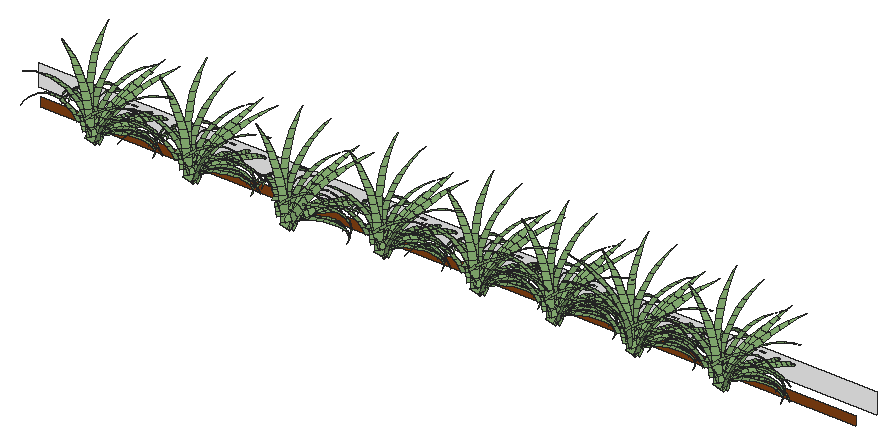
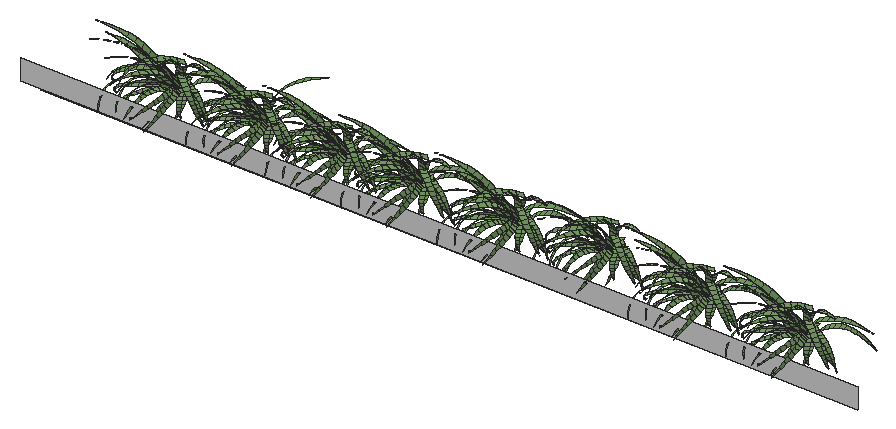
# SketchUp Ruby script. Lengths in inches.
U = 1.inch
M = Sketchup.active_model
def pt(a) = Geom::Point3d.new(a.map { |v| v * U })
def face(e, loops, mat)
  f = e.add_face(loops[0].map { |a| pt(a) })
  loops[1..].each { |l| e.add_face(l.map { |a| pt(a) }).erase! }
  f.material = f.back_material = mat if mat
  f
end
# faces: each face lists its corners as indices into pts; further lists are holes
def faces(e, pts, list, mat = nil) = list.each { |f| face(e, (f[0].is_a?(Array) ? f : [f]).map { |l| l.map { |i| pts[i] } }, mat) }
# xy, xz, yz: faces in a plane at the given z, y or x. An outline is a flat list of corners, or four numbers for a rectangle; further outlines are holes
def ring(l) = l.size == 4 ? [[l[0], l[1]], [l[2], l[1]], [l[2], l[3]], [l[0], l[3]]] : l.each_slice(2).to_a
def flat(e, list, mat, &to3) = list.each { |f| face(e, (f[0].is_a?(Array) ? f : [f]).map { |l| ring(l).map { |u, v| to3.(u, v) } }, mat) }
def xy(e, z, list, mat = nil) = flat(e, list, mat) { |x, y| [x, y, z] }
def xz(e, y, list, mat = nil) = flat(e, list, mat) { |x, z| [x, y, z] }
def yz(e, x, list, mat = nil) = flat(e, list, mat) { |y, z| [x, y, z] }
def lines(e, pts, list) = list.each { |a, b| e.add_line(pt(pts[a]), pt(pts[b])) }
# prism: a flat outline (further loops are holes) pulled along v
def prism(e, loops, v, mat = nil)
  f = face(e, loops, mat); d = Geom::Vector3d.new(v.map { |x| x * U })
  f.pushpull(f.normal.samedirection?(d) ? d.length : -d.length)
end
def box(e, o, s, mat = nil) = prism(e, [[o, [o[0] + s[0], o[1], o[2]], [o[0] + s[0], o[1] + s[1], o[2]], [o[0], o[1] + s[1], o[2]]]], [0, 0, s[2]], mat)
def at(x, y, z, deg = 0) = Geom::Transformation.translation(pt([x, y, z])) * Geom::Transformation.rotation(ORIGIN, Z_AXIS, deg.degrees)
def axes(o, x, y, z) = Geom::Transformation.new([*x, 0, *y, 0, *z, 0, *pt(o).to_a, 1])
def part(name) = M.definitions.add(name)
# library, detail: a bought-in or finely detailed component or shape, given as its bounding box
def library(name, o, s) = part(name).tap { |d| box(d.entities, o, s) }
def detail(e, o, s) = box(e.add_group.entities, o, s)
def put(e, d, t, mat = nil) = e.add_instance(d, t).tap { |i| i.material = mat if mat }
def group(e, t, mat = nil) = e.add_group.tap { |g| g.transformation = t; g.material = mat if mat }.entities
root = M.entities
M.materials.add("[0043_SaddleBrown]").color = [139, 69, 19]
M.materials.add("[Color M00]").color = [255, 255, 255]
M.materials.add("dianella").color = [131, 171, 111]
c1 = part("Shape Bender Component\#7")
p = [[0.01,0.94,1.17],[0.04,0.96,6.32],[0.04,4.67,6.32],[0.01,4.68,1.17],[0.42,0.98,10.52],[0.51,1,11.45],
  [0.51,4.64,11.45],[0.42,4.66,10.52],[1.4,1.07,16.52],[1.4,4.57,16.52],[2.48,1.13,20.62],[2.71,1.16,21.49],
  [2.71,4.49,21.49],[2.48,4.52,20.625],[4.4375,1.21,26.32],[4.4375,4.46,26.32],[6.56,1.22,30.98],[6.56,4.47,30.98],
  [9.06,1.29,35.43],[9.06,4.38,35.43],[11.92,1.42,39.64],[11.92,4.23,39.64],[15.13,1.74,43.57],[15.13,4,43.57],
  [18.65,2.08,47.2],[18.65,3.67,47.2],[22.46,2.47,50.5],[22.46,3.14,50.5],[25.84,2.81,52.95]]
faces(c1.entities,p,[[0,1,2,3],[1,4,5,6,7,2],[5,8,9,6],[10,11,12,13,9,8],[11,14,15,12],[14,16,17,15],[16,18,19,17],[18,20,21,19],
  [20,22,23,21],[22,24,25,23],[24,26,27,25],[28,27,26]],"dianella")
c2 = part("Shape Bender Component\#4")
p = [[0.27,1.78,0.46],[1.95,1.8,3.35],[1.95,4.67,3.35],[0.27,4.68,0.46],[3.06,1.81,4.8],[3.875,1.84,5.87],
  [3.875,4.64,5.87],[3.06,4.66,4.8],[6,1.9,8],[6,4.58,8],[27.35,3.23,6.09],[25.57,3.4375,7.9],
  [25.57,3.03,7.9],[23.28,2.8,9.61],[23.28,3.67,9.61],[7.08,1.93,8.8],[8.3,1.99,9.69],[8.3,4.5,9.69],
  [7.08,4.55,8.8],[23.04,2.78,9.74],[23.04,3.69,9.74],[20.86,3.86,10.86],[20.86,2.625,10.86],[10.73,2.08,10.92],
  [10.73,4.41,10.92],[12.13,2.13,11.33],[13.24,2.19,11.66],[13.24,4.3,11.66],[12.13,4.36,11.33],[18.35,2.46,11.63],
  [18.35,4.03,11.63],[15.79,2.32,11.89],[17.75,2.42,11.69],[17.75,4.07,11.69],[15.79,4.17,11.89]]
faces(c2.entities,p,[[0,1,2,3],[1,4,5,6,7,2],[5,8,9,6],[10,11,12],[13,12,11,14],[15,16,17,18,9,8],[19,13,14,20,21,22],[16,23,24,17],
  [23,25,26,27,28,24],[29,22,21,30],[31,32,29,30,33,34],[26,31,34,27]],"dianella")
c3 = part("Shape Bender Component\#5")
p = [[0.17,0.01,0.72],[1.09,0.03,4.5625],[1.09,3.73,4.5625],[0.17,3.75,0.72],[2.23,0.05,7.59],[2.48,0.0625,8.26],
  [2.48,3.71,8.26],[2.23,3.72,7.59],[4.33,0.14,11.74],[4.33,3.64,11.74],[6.2,0.2,14.41],[6.6,0.22,14.97],
  [6.6,3.56,14.97],[6.2,3.58,14.41],[9.26,0.35,17.88],[9.26,3.43,17.88],[12.27,0.4,20.43],[12.27,3.38,20.43],
  [15.58,0.51,22.59],[15.58,3.27,22.59],[19.13,0.73,24.3],[19.13,3.14,24.3],[22.875,1.08,25.56],[22.875,2.85,25.56],
  [26.75,1.47,26.33],[26.75,2.49,26.33],[30.68,1.86,26.6],[30.68,2.125,26.6],[33.95,1.875,26.45]]
faces(c3.entities,p,[[0,1,2,3],[1,4,5,6,7,2],[5,8,9,6],[8,10,11,12,13,9],[11,14,15,12],[14,16,17,15],[16,18,19,17],[18,20,21,19],
  [20,22,23,21],[22,24,25,23],[24,26,27,25],[28,27,26]],"dianella")
xz(root,570,[[30,281.8125,450,286.25]],"[0043_SaddleBrown]")
xz(root,576,[[24,286.25,456,297.0625]],"[Color M00]")
put(root,c1,axes([351.64,546.07,292.41],[-0.96457,-0.17955,-0.21457],[-0.1415,0.96983,-0.21622],[-0.14686,0.09469,0.71579]))
put(root,c2,axes([116.66,547.22,296.58],[-0.96457,-0.17955,-0.21457],[-0.12461,0.95587,-0.29533],[-0.20696,0.20696,0.93295]))
put(root,c2,axes([215.07,547.22,296.58],[-0.96457,-0.17955,-0.21457],[-0.12461,0.95587,-0.29533],[-0.20696,0.20696,0.93295]))
put(root,c2,axes([303.54,547.22,296.58],[-0.96457,-0.17955,-0.21457],[-0.12461,0.95587,-0.29533],[-0.20696,0.20696,0.93295]))
put(root,c2,axes([389.75,547.22,296.58],[-0.96457,-0.17955,-0.21457],[-0.12461,0.95587,-0.29533],[-0.20696,0.20696,0.93295]))
put(root,c2,axes([66.14,547.22,296.58],[-0.96457,-0.17955,-0.21457],[-0.12461,0.95587,-0.29533],[-0.20696,0.20696,0.93295]))
put(root,c2,axes([264.63,547.22,296.58],[-0.96457,-0.17955,-0.21457],[-0.12461,0.95587,-0.29533],[-0.20696,0.20696,0.93295]))
put(root,c2,axes([344.64,547.22,296.58],[-0.96457,-0.17955,-0.21457],[-0.12461,0.95587,-0.29533],[-0.20696,0.20696,0.93295]))
put(root,c2,axes([180,535.97,302.54],[0.64426,0.58365,-0.4226],[-0.74526,0.62305,-0.21648],[0.16818,0.5202,0.75394]))
put(root,c3,axes([122.69,550.63,289.92],[0.94077,-0.2561,-0.22218],[0.2011,0.94909,-0.24247],[0.24294,0.16325,0.84049]))
put(root,c3,axes([221.1,550.63,289.92],[0.94077,-0.2561,-0.22218],[0.2011,0.94909,-0.24247],[0.24294,0.16325,0.84049]))
put(root,c3,axes([309.57,550.63,289.92],[0.94077,-0.2561,-0.22218],[0.2011,0.94909,-0.24247],[0.24294,0.16325,0.84049]))
put(root,c3,axes([395.78,550.63,289.92],[0.94077,-0.2561,-0.22218],[0.2011,0.94909,-0.24247],[0.24294,0.16325,0.84049]))
put(root,c3,axes([72.17,550.63,289.92],[0.94077,-0.2561,-0.22218],[0.2011,0.94909,-0.24247],[0.24294,0.16325,0.84049]))
put(root,c3,axes([270.66,550.63,289.92],[0.94077,-0.2561,-0.22218],[0.2011,0.94909,-0.24247],[0.24294,0.16325,0.84049]))
put(root,c3,axes([350.67,550.63,289.92],[0.94077,-0.2561,-0.22218],[0.2011,0.94909,-0.24247],[0.24294,0.16325,0.84049]))
put(root,c2,axes([184.96,543.86,301.61],[0.57501,0.09261,-0.46633],[-0.47395,0.84751,-0.13449],[0.65517,0.51591,0.262]))
put(root,c3,axes([123.37,548.09,291.63],[-0.97248,-0.07019,-0.24662],[-0.01462,0.97005,-0.26914],[-0.20696,0.20696,0.93295]))
put(root,c3,axes([221.77,548.09,291.63],[-0.97248,-0.07019,-0.24662],[-0.01462,0.97005,-0.26914],[-0.20696,0.20696,0.93295]))
put(root,c3,axes([310.25,548.09,291.63],[-0.97248,-0.07019,-0.24662],[-0.01462,0.97005,-0.26914],[-0.20696,0.20696,0.93295]))
put(root,c3,axes([396.45,548.09,291.63],[-0.97248,-0.07019,-0.24662],[-0.01462,0.97005,-0.26914],[-0.20696,0.20696,0.93295]))
put(root,c3,axes([72.84,548.09,291.63],[-0.97248,-0.07019,-0.24662],[-0.01462,0.97005,-0.26914],[-0.20696,0.20696,0.93295]))
put(root,c3,axes([271.33,548.09,291.63],[-0.97248,-0.07019,-0.24662],[-0.01462,0.97005,-0.26914],[-0.20696,0.20696,0.93295]))
put(root,c3,axes([351.34,548.09,291.63],[-0.97248,-0.07019,-0.24662],[-0.01462,0.97005,-0.26914],[-0.20696,0.20696,0.93295]))
put(root,c2,axes([183.52,544.4,294.32],[0.57501,0.09261,-0.31801],[-0.47395,0.84751,-0.09172],[0.65517,0.51591,0.17867]))
put(root,c1,axes([175.95,540.82,291.04],[-0.8536,0.41658,-0.34718],[0.46614,0.87885,-0.1128],[-0.15322,0.15322,0.69068]))
put(root,c2,axes([171.79,543.85,295.76],[-0.8536,0.41658,-0.34718],[0.46614,0.87885,-0.1128],[-0.20696,0.20696,0.93295]))
put(root,c2,axes([168.27,544.69,300.99],[-0.54643,0.20158,-0.353],[0.62824,0.74041,-0.10181],[-0.54359,0.63239,0.19832]))
put(root,c2,axes([173.8125,539.64,293.97],[-0.37814,0.80953,-0.24696],[0.77879,0.53846,0.16717],[-0.48914,0.20852,0.40507]))
put(root,c2,axes([182.12,541.8,293.25],[0.43451,0.44271,-0.29722],[-0.79952,0.58659,-0.03391],[0.39557,0.673,0.20362]))
put(root,c3,axes([126.78,546.74,291.2],[0.98276,0.1646,0.08419],[-0.14484,0.96332,-0.19265],[-0.10945,0.21065,0.86584]))
put(root,c3,axes([225.1875,546.74,291.2],[0.98276,0.1646,0.08419],[-0.14484,0.96332,-0.19265],[-0.10945,0.21065,0.86584]))
put(root,c3,axes([313.66,546.74,291.2],[0.98276,0.1646,0.08419],[-0.14484,0.96332,-0.19265],[-0.10945,0.21065,0.86584]))
put(root,c3,axes([399.87,546.74,291.2],[0.98276,0.1646,0.08419],[-0.14484,0.96332,-0.19265],[-0.10945,0.21065,0.86584]))
put(root,c3,axes([76.26,546.74,291.2],[0.98276,0.1646,0.08419],[-0.14484,0.96332,-0.19265],[-0.10945,0.21065,0.86584]))
put(root,c3,axes([274.75,546.74,291.2],[0.98276,0.1646,0.08419],[-0.14484,0.96332,-0.19265],[-0.10945,0.21065,0.86584]))
put(root,c3,axes([354.76,546.74,291.2],[0.98276,0.1646,0.08419],[-0.14484,0.96332,-0.19265],[-0.10945,0.21065,0.86584]))
put(root,c2,axes([127.29,547.1,293.64],[0.91783,0.24445,-0.31277],[-0.28823,0.95215,-0.10163],[0.24294,0.16325,0.84049]))
put(root,c2,axes([225.69,547.1,293.64],[0.91783,0.24445,-0.31277],[-0.28823,0.95215,-0.10163],[0.24294,0.16325,0.84049]))
put(root,c2,axes([314.17,547.1,293.64],[0.91783,0.24445,-0.31277],[-0.28823,0.95215,-0.10163],[0.24294,0.16325,0.84049]))
put(root,c2,axes([400.37,547.1,293.64],[0.91783,0.24445,-0.31277],[-0.28823,0.95215,-0.10163],[0.24294,0.16325,0.84049]))
put(root,c2,axes([76.77,547.1,293.64],[0.91783,0.24445,-0.31277],[-0.28823,0.95215,-0.10163],[0.24294,0.16325,0.84049]))
put(root,c2,axes([275.25,547.1,293.64],[0.91783,0.24445,-0.31277],[-0.28823,0.95215,-0.10163],[0.24294,0.16325,0.84049]))
put(root,c2,axes([355.26,547.1,293.64],[0.91783,0.24445,-0.31277],[-0.28823,0.95215,-0.10163],[0.24294,0.16325,0.84049]))
put(root,c2,axes([169.14,541.87,299.79],[-0.34116,0.51808,-0.32991],[0.89749,0.4217,-0.03764],[-0.25861,0.73656,0.22602]))
put(root,c2,axes([125.52,541.97,302.54],[0.64426,0.58365,-0.4226],[-0.74526,0.62305,-0.21648],[0.16818,0.5202,0.75394]))
put(root,c2,axes([223.92,541.97,302.54],[0.64426,0.58365,-0.4226],[-0.74526,0.62305,-0.21648],[0.16818,0.5202,0.75394]))
put(root,c2,axes([312.4,541.97,302.54],[0.64426,0.58365,-0.4226],[-0.74526,0.62305,-0.21648],[0.16818,0.5202,0.75394]))
put(root,c2,axes([398.6,541.97,302.54],[0.64426,0.58365,-0.4226],[-0.74526,0.62305,-0.21648],[0.16818,0.5202,0.75394]))
put(root,c2,axes([75,541.97,302.54],[0.64426,0.58365,-0.4226],[-0.74526,0.62305,-0.21648],[0.16818,0.5202,0.75394]))
put(root,c2,axes([273.48,541.97,302.54],[0.64426,0.58365,-0.4226],[-0.74526,0.62305,-0.21648],[0.16818,0.5202,0.75394]))
put(root,c2,axes([353.49,541.97,302.54],[0.64426,0.58365,-0.4226],[-0.74526,0.62305,-0.21648],[0.16818,0.5202,0.75394]))
put(root,c2,axes([169.1875,547.18,304.6],[-0.54643,0.20158,-0.51762],[0.62824,0.74041,-0.14929],[-0.54359,0.63239,0.29082]))
put(root,c2,axes([178.9,541.9,290.9375],[0.19337,0.9127,-0.35512],[-0.68492,0.38442,0.57846],[0.69138,0.1105,0.59486]))
put(root,c2,axes([130.48,549.86,301.61],[0.57501,0.09261,-0.46633],[-0.47395,0.84751,-0.13449],[0.65517,0.51591,0.262]))
put(root,c2,axes([228.88,549.86,301.61],[0.57501,0.09261,-0.46633],[-0.47395,0.84751,-0.13449],[0.65517,0.51591,0.262]))
put(root,c2,axes([317.36,549.86,301.61],[0.57501,0.09261,-0.46633],[-0.47395,0.84751,-0.13449],[0.65517,0.51591,0.262]))
put(root,c2,axes([403.56,549.86,301.61],[0.57501,0.09261,-0.46633],[-0.47395,0.84751,-0.13449],[0.65517,0.51591,0.262]))
put(root,c2,axes([79.96,549.86,301.61],[0.57501,0.09261,-0.46633],[-0.47395,0.84751,-0.13449],[0.65517,0.51591,0.262]))
put(root,c2,axes([278.44,549.86,301.61],[0.57501,0.09261,-0.46633],[-0.47395,0.84751,-0.13449],[0.65517,0.51591,0.262]))
put(root,c2,axes([358.45,549.86,301.61],[0.57501,0.09261,-0.46633],[-0.47395,0.84751,-0.13449],[0.65517,0.51591,0.262]))
put(root,c2,axes([181.62,542.72,288.01],[0.00951,0.98109,-0.1933],[-0.96198,0.06174,0.26606],[0.24294,0.16325,0.84049]))
put(root,c2,axes([129.04,550.4,294.32],[0.57501,0.09261,-0.31801],[-0.47395,0.84751,-0.09172],[0.65517,0.51591,0.17867]))
put(root,c2,axes([227.44,550.4,294.32],[0.57501,0.09261,-0.31801],[-0.47395,0.84751,-0.09172],[0.65517,0.51591,0.17867]))
put(root,c2,axes([315.92,550.4,294.32],[0.57501,0.09261,-0.31801],[-0.47395,0.84751,-0.09172],[0.65517,0.51591,0.17867]))
put(root,c2,axes([402.125,550.4,294.32],[0.57501,0.09261,-0.31801],[-0.47395,0.84751,-0.09172],[0.65517,0.51591,0.17867]))
put(root,c2,axes([78.52,550.4,294.32],[0.57501,0.09261,-0.31801],[-0.47395,0.84751,-0.09172],[0.65517,0.51591,0.17867]))
put(root,c2,axes([277,550.4,294.32],[0.57501,0.09261,-0.31801],[-0.47395,0.84751,-0.09172],[0.65517,0.51591,0.17867]))
put(root,c2,axes([357.01,550.4,294.32],[0.57501,0.09261,-0.31801],[-0.47395,0.84751,-0.09172],[0.65517,0.51591,0.17867]))
put(root,c1,axes([180.08,542.89,287.55],[0.29029,0.93027,-0.22347],[-0.88563,0.34788,0.30262],[0.28937,0.069,0.69734]))
put(root,c1,axes([121.47,546.82,291.04],[-0.8536,0.41658,-0.34718],[0.46614,0.87885,-0.1128],[-0.15322,0.15322,0.69068]))
put(root,c1,axes([219.87,546.82,291.04],[-0.8536,0.41658,-0.34718],[0.46614,0.87885,-0.1128],[-0.15322,0.15322,0.69068]))
put(root,c1,axes([308.35,546.82,291.04],[-0.8536,0.41658,-0.34718],[0.46614,0.87885,-0.1128],[-0.15322,0.15322,0.69068]))
put(root,c1,axes([394.55,546.82,291.04],[-0.8536,0.41658,-0.34718],[0.46614,0.87885,-0.1128],[-0.15322,0.15322,0.69068]))
put(root,c1,axes([70.95,546.82,291.04],[-0.8536,0.41658,-0.34718],[0.46614,0.87885,-0.1128],[-0.15322,0.15322,0.69068]))
put(root,c1,axes([269.43,546.82,291.04],[-0.8536,0.41658,-0.34718],[0.46614,0.87885,-0.1128],[-0.15322,0.15322,0.69068]))
put(root,c1,axes([349.44,546.82,291.04],[-0.8536,0.41658,-0.34718],[0.46614,0.87885,-0.1128],[-0.15322,0.15322,0.69068]))
put(root,c2,axes([174.76,544.09,292.76],[-0.01403,0.93285,-0.39418],[0.74612,0.24536,0.64209],[-0.65717,0.24154,0.6603]))
put(root,c2,axes([117.3,549.85,295.76],[-0.8536,0.41658,-0.34718],[0.46614,0.87885,-0.1128],[-0.20696,0.20696,0.93295]))
put(root,c2,axes([215.71,549.85,295.76],[-0.8536,0.41658,-0.34718],[0.46614,0.87885,-0.1128],[-0.20696,0.20696,0.93295]))
put(root,c2,axes([304.1875,549.85,295.76],[-0.8536,0.41658,-0.34718],[0.46614,0.87885,-0.1128],[-0.20696,0.20696,0.93295]))
put(root,c2,axes([390.39,549.85,295.76],[-0.8536,0.41658,-0.34718],[0.46614,0.87885,-0.1128],[-0.20696,0.20696,0.93295]))
put(root,c2,axes([66.78,549.85,295.76],[-0.8536,0.41658,-0.34718],[0.46614,0.87885,-0.1128],[-0.20696,0.20696,0.93295]))
put(root,c2,axes([265.27,549.85,295.76],[-0.8536,0.41658,-0.34718],[0.46614,0.87885,-0.1128],[-0.20696,0.20696,0.93295]))
put(root,c2,axes([345.28,549.85,295.76],[-0.8536,0.41658,-0.34718],[0.46614,0.87885,-0.1128],[-0.20696,0.20696,0.93295]))
put(root,c2,axes([113.78,550.69,300.99],[-0.54643,0.20158,-0.353],[0.62824,0.74041,-0.10181],[-0.54359,0.63239,0.19832]))
put(root,c2,axes([212.1875,550.69,300.99],[-0.54643,0.20158,-0.353],[0.62824,0.74041,-0.10181],[-0.54359,0.63239,0.19832]))
put(root,c2,axes([300.66,550.69,300.99],[-0.54643,0.20158,-0.353],[0.62824,0.74041,-0.10181],[-0.54359,0.63239,0.19832]))
put(root,c2,axes([386.87,550.69,300.99],[-0.54643,0.20158,-0.353],[0.62824,0.74041,-0.10181],[-0.54359,0.63239,0.19832]))
put(root,c2,axes([63.26,550.69,300.99],[-0.54643,0.20158,-0.353],[0.62824,0.74041,-0.10181],[-0.54359,0.63239,0.19832]))
put(root,c2,axes([261.75,550.69,300.99],[-0.54643,0.20158,-0.353],[0.62824,0.74041,-0.10181],[-0.54359,0.63239,0.19832]))
put(root,c2,axes([341.76,550.69,300.99],[-0.54643,0.20158,-0.353],[0.62824,0.74041,-0.10181],[-0.54359,0.63239,0.19832]))
put(root,c2,axes([119.33,545.64,293.97],[-0.37814,0.80953,-0.24696],[0.77879,0.53846,0.16717],[-0.48914,0.20852,0.40507]))
put(root,c2,axes([217.73,545.64,293.97],[-0.37814,0.80953,-0.24696],[0.77879,0.53846,0.16717],[-0.48914,0.20852,0.40507]))
put(root,c2,axes([306.21,545.64,293.97],[-0.37814,0.80953,-0.24696],[0.77879,0.53846,0.16717],[-0.48914,0.20852,0.40507]))
put(root,c2,axes([392.41,545.64,293.97],[-0.37814,0.80953,-0.24696],[0.77879,0.53846,0.16717],[-0.48914,0.20852,0.40507]))
put(root,c2,axes([68.81,545.64,293.97],[-0.37814,0.80953,-0.24696],[0.77879,0.53846,0.16717],[-0.48914,0.20852,0.40507]))
put(root,c2,axes([267.29,545.64,293.97],[-0.37814,0.80953,-0.24696],[0.77879,0.53846,0.16717],[-0.48914,0.20852,0.40507]))
put(root,c2,axes([347.3,545.64,293.97],[-0.37814,0.80953,-0.24696],[0.77879,0.53846,0.16717],[-0.48914,0.20852,0.40507]))
put(root,c2,axes([127.63,547.8,293.25],[0.43451,0.44271,-0.29722],[-0.79952,0.58659,-0.03391],[0.39557,0.673,0.20362]))
put(root,c2,axes([226.04,547.8,293.25],[0.43451,0.44271,-0.29722],[-0.79952,0.58659,-0.03391],[0.39557,0.673,0.20362]))
put(root,c2,axes([314.51,547.8,293.25],[0.43451,0.44271,-0.29722],[-0.79952,0.58659,-0.03391],[0.39557,0.673,0.20362]))
put(root,c2,axes([400.72,547.8,293.25],[0.43451,0.44271,-0.29722],[-0.79952,0.58659,-0.03391],[0.39557,0.673,0.20362]))
put(root,c2,axes([77.11,547.8,293.25],[0.43451,0.44271,-0.29722],[-0.79952,0.58659,-0.03391],[0.39557,0.673,0.20362]))
put(root,c2,axes([275.6,547.8,293.25],[0.43451,0.44271,-0.29722],[-0.79952,0.58659,-0.03391],[0.39557,0.673,0.20362]))
put(root,c2,axes([355.61,547.8,293.25],[0.43451,0.44271,-0.29722],[-0.79952,0.58659,-0.03391],[0.39557,0.673,0.20362]))
put(root,c2,axes([183,545.71,291.44],[0.00951,0.98109,-0.1933],[-0.71163,0.13509,0.65066],[0.69138,0.1105,0.59486]))
put(root,c1,axes([181.62,544.44,287.67],[0.00951,0.98109,-0.1933],[-0.96198,0.06174,0.26606],[0.1822,0.12244,0.63037]))
put(root,c2,axes([174.41,546.42,289.51],[0.17955,0.96457,-0.21457],[0.95587,-0.12461,0.29533],[-0.20696,0.20696,0.93295]))
put(root,c2,axes([114.66,547.87,299.79],[-0.34116,0.51808,-0.32991],[0.89749,0.4217,-0.03764],[-0.25861,0.73656,0.22602]))
put(root,c2,axes([213.07,547.87,299.79],[-0.34116,0.51808,-0.32991],[0.89749,0.4217,-0.03764],[-0.25861,0.73656,0.22602]))
put(root,c2,axes([301.54,547.87,299.79],[-0.34116,0.51808,-0.32991],[0.89749,0.4217,-0.03764],[-0.25861,0.73656,0.22602]))
put(root,c2,axes([387.75,547.87,299.79],[-0.34116,0.51808,-0.32991],[0.89749,0.4217,-0.03764],[-0.25861,0.73656,0.22602]))
put(root,c2,axes([64.14,547.87,299.79],[-0.34116,0.51808,-0.32991],[0.89749,0.4217,-0.03764],[-0.25861,0.73656,0.22602]))
put(root,c2,axes([262.625,547.87,299.79],[-0.34116,0.51808,-0.32991],[0.89749,0.4217,-0.03764],[-0.25861,0.73656,0.22602]))
put(root,c2,axes([342.64,547.87,299.79],[-0.34116,0.51808,-0.32991],[0.89749,0.4217,-0.03764],[-0.25861,0.73656,0.22602]))
put(root,c1,axes([173.79,545.28,289],[-0.10576,0.96875,-0.24806],[0.93604,0.17087,0.33591],[-0.27067,0.12342,0.77405]))
put(root,c3,axes([178.19,542.87,288.69],[-0.09945,0.98178,-0.16194],[-0.95687,-0.04972,0.28623],[0.24294,0.16325,0.84049]))
put(root,c2,axes([186.44,547.68,294.24],[0.19337,0.9127,-0.35512],[-0.68492,0.38442,0.57846],[0.69138,0.1105,0.59486]))
put(root,c2,axes([114.7,553.18,304.6],[-0.54643,0.20158,-0.51762],[0.62824,0.74041,-0.14929],[-0.54359,0.63239,0.29082]))
put(root,c2,axes([213.11,553.18,304.6],[-0.54643,0.20158,-0.51762],[0.62824,0.74041,-0.14929],[-0.54359,0.63239,0.29082]))
put(root,c2,axes([301.59,553.18,304.6],[-0.54643,0.20158,-0.51762],[0.62824,0.74041,-0.14929],[-0.54359,0.63239,0.29082]))
put(root,c2,axes([387.79,553.18,304.6],[-0.54643,0.20158,-0.51762],[0.62824,0.74041,-0.14929],[-0.54359,0.63239,0.29082]))
put(root,c2,axes([64.18,553.18,304.6],[-0.54643,0.20158,-0.51762],[0.62824,0.74041,-0.14929],[-0.54359,0.63239,0.29082]))
put(root,c2,axes([262.67,553.18,304.6],[-0.54643,0.20158,-0.51762],[0.62824,0.74041,-0.14929],[-0.54359,0.63239,0.29082]))
put(root,c2,axes([342.68,553.18,304.6],[-0.54643,0.20158,-0.51762],[0.62824,0.74041,-0.14929],[-0.54359,0.63239,0.29082]))
put(root,c2,axes([124.41,547.9,290.9375],[0.19337,0.9127,-0.35512],[-0.68492,0.38442,0.57846],[0.69138,0.1105,0.59486]))
put(root,c2,axes([222.82,547.9,290.9375],[0.19337,0.9127,-0.35512],[-0.68492,0.38442,0.57846],[0.69138,0.1105,0.59486]))
put(root,c2,axes([311.29,547.9,290.9375],[0.19337,0.9127,-0.35512],[-0.68492,0.38442,0.57846],[0.69138,0.1105,0.59486]))
put(root,c2,axes([397.5,547.9,290.9375],[0.19337,0.9127,-0.35512],[-0.68492,0.38442,0.57846],[0.69138,0.1105,0.59486]))
put(root,c2,axes([73.89,547.9,290.9375],[0.19337,0.9127,-0.35512],[-0.68492,0.38442,0.57846],[0.69138,0.1105,0.59486]))
put(root,c2,axes([272.38,547.9,290.9375],[0.19337,0.9127,-0.35512],[-0.68492,0.38442,0.57846],[0.69138,0.1105,0.59486]))
put(root,c2,axes([352.39,547.9,290.9375],[0.19337,0.9127,-0.35512],[-0.68492,0.38442,0.57846],[0.69138,0.1105,0.59486]))
put(root,c3,axes([175.64,544.9,290.26],[0.28661,0.94426,-0.17976],[0.9294,-0.23301,0.31772],[-0.20696,0.20696,0.93295]))
put(root,c2,axes([171.47,548.61,293.3125],[0.17955,0.96457,-0.21457],[0.72432,-0.00444,0.72223],[-0.65717,0.24154,0.6603]))
put(root,c1,axes([172.58,547.1,289.13],[0.17955,0.96457,-0.21457],[0.95587,-0.12461,0.29533],[-0.15522,0.15522,0.69971]))
put(root,c2,axes([127.13,548.72,288.01],[0.00951,0.98109,-0.1933],[-0.96198,0.06174,0.26606],[0.24294,0.16325,0.84049]))
put(root,c2,axes([225.54,548.72,288.01],[0.00951,0.98109,-0.1933],[-0.96198,0.06174,0.26606],[0.24294,0.16325,0.84049]))
put(root,c2,axes([314.02,548.72,288.01],[0.00951,0.98109,-0.1933],[-0.96198,0.06174,0.26606],[0.24294,0.16325,0.84049]))
put(root,c2,axes([400.22,548.72,288.01],[0.00951,0.98109,-0.1933],[-0.96198,0.06174,0.26606],[0.24294,0.16325,0.84049]))
put(root,c2,axes([76.61,548.72,288.01],[0.00951,0.98109,-0.1933],[-0.96198,0.06174,0.26606],[0.24294,0.16325,0.84049]))
put(root,c2,axes([275.1,548.72,288.01],[0.00951,0.98109,-0.1933],[-0.96198,0.06174,0.26606],[0.24294,0.16325,0.84049]))
put(root,c2,axes([355.11,548.72,288.01],[0.00951,0.98109,-0.1933],[-0.96198,0.06174,0.26606],[0.24294,0.16325,0.84049]))
put(root,c1,axes([125.59,548.89,287.55],[0.29029,0.93027,-0.22347],[-0.88563,0.34788,0.30262],[0.28937,0.069,0.69734]))
put(root,c1,axes([224,548.89,287.55],[0.29029,0.93027,-0.22347],[-0.88563,0.34788,0.30262],[0.28937,0.069,0.69734]))
put(root,c1,axes([312.47,548.89,287.55],[0.29029,0.93027,-0.22347],[-0.88563,0.34788,0.30262],[0.28937,0.069,0.69734]))
put(root,c1,axes([398.68,548.89,287.55],[0.29029,0.93027,-0.22347],[-0.88563,0.34788,0.30262],[0.28937,0.069,0.69734]))
put(root,c1,axes([75.07,548.89,287.55],[0.29029,0.93027,-0.22347],[-0.88563,0.34788,0.30262],[0.28937,0.069,0.69734]))
put(root,c1,axes([273.56,548.89,287.55],[0.29029,0.93027,-0.22347],[-0.88563,0.34788,0.30262],[0.28937,0.069,0.69734]))
put(root,c1,axes([353.57,548.89,287.55],[0.29029,0.93027,-0.22347],[-0.88563,0.34788,0.30262],[0.28937,0.069,0.69734]))
put(root,c2,axes([120.28,550.09,292.76],[-0.01403,0.93285,-0.39418],[0.74612,0.24536,0.64209],[-0.65717,0.24154,0.6603]))
put(root,c2,axes([218.68,550.09,292.76],[-0.01403,0.93285,-0.39418],[0.74612,0.24536,0.64209],[-0.65717,0.24154,0.6603]))
put(root,c2,axes([307.16,550.09,292.76],[-0.01403,0.93285,-0.39418],[0.74612,0.24536,0.64209],[-0.65717,0.24154,0.6603]))
put(root,c2,axes([393.36,550.09,292.76],[-0.01403,0.93285,-0.39418],[0.74612,0.24536,0.64209],[-0.65717,0.24154,0.6603]))
put(root,c2,axes([69.76,550.09,292.76],[-0.01403,0.93285,-0.39418],[0.74612,0.24536,0.64209],[-0.65717,0.24154,0.6603]))
put(root,c2,axes([268.24,550.09,292.76],[-0.01403,0.93285,-0.39418],[0.74612,0.24536,0.64209],[-0.65717,0.24154,0.6603]))
put(root,c2,axes([348.25,550.09,292.76],[-0.01403,0.93285,-0.39418],[0.74612,0.24536,0.64209],[-0.65717,0.24154,0.6603]))
put(root,c2,axes([128.52,551.71,291.44],[0.00951,0.98109,-0.1933],[-0.71163,0.13509,0.65066],[0.69138,0.1105,0.59486]))
put(root,c2,axes([226.92,551.71,291.44],[0.00951,0.98109,-0.1933],[-0.71163,0.13509,0.65066],[0.69138,0.1105,0.59486]))
put(root,c2,axes([315.4,551.71,291.44],[0.00951,0.98109,-0.1933],[-0.71163,0.13509,0.65066],[0.69138,0.1105,0.59486]))
put(root,c2,axes([401.6,551.71,291.44],[0.00951,0.98109,-0.1933],[-0.71163,0.13509,0.65066],[0.69138,0.1105,0.59486]))
put(root,c2,axes([77.99,551.71,291.44],[0.00951,0.98109,-0.1933],[-0.71163,0.13509,0.65066],[0.69138,0.1105,0.59486]))
put(root,c2,axes([276.48,551.71,291.44],[0.00951,0.98109,-0.1933],[-0.71163,0.13509,0.65066],[0.69138,0.1105,0.59486]))
put(root,c2,axes([356.49,551.71,291.44],[0.00951,0.98109,-0.1933],[-0.71163,0.13509,0.65066],[0.69138,0.1105,0.59486]))
put(root,c2,axes([168.47,551.21,296.42],[-0.01403,0.93285,-0.39418],[0.74612,0.24536,0.64209],[-0.65717,0.24154,0.6603]))
put(root,c1,axes([127.13,550.44,287.67],[0.00951,0.98109,-0.1933],[-0.96198,0.06174,0.26606],[0.1822,0.12244,0.63037]))
put(root,c1,axes([225.54,550.44,287.67],[0.00951,0.98109,-0.1933],[-0.96198,0.06174,0.26606],[0.1822,0.12244,0.63037]))
put(root,c1,axes([314.01,550.44,287.67],[0.00951,0.98109,-0.1933],[-0.96198,0.06174,0.26606],[0.1822,0.12244,0.63037]))
put(root,c1,axes([400.22,550.44,287.67],[0.00951,0.98109,-0.1933],[-0.96198,0.06174,0.26606],[0.1822,0.12244,0.63037]))
put(root,c1,axes([76.61,550.44,287.67],[0.00951,0.98109,-0.1933],[-0.96198,0.06174,0.26606],[0.1822,0.12244,0.63037]))
put(root,c1,axes([275.1,550.44,287.67],[0.00951,0.98109,-0.1933],[-0.96198,0.06174,0.26606],[0.1822,0.12244,0.63037]))
put(root,c1,axes([355.11,550.44,287.67],[0.00951,0.98109,-0.1933],[-0.96198,0.06174,0.26606],[0.1822,0.12244,0.63037]))
put(root,c2,axes([119.92,552.42,289.51],[0.17955,0.96457,-0.21457],[0.95587,-0.12461,0.29533],[-0.20696,0.20696,0.93295]))
put(root,c2,axes([218.33,552.42,289.51],[0.17955,0.96457,-0.21457],[0.95587,-0.12461,0.29533],[-0.20696,0.20696,0.93295]))
put(root,c2,axes([306.8,552.42,289.51],[0.17955,0.96457,-0.21457],[0.95587,-0.12461,0.29533],[-0.20696,0.20696,0.93295]))
put(root,c2,axes([393.01,552.42,289.51],[0.17955,0.96457,-0.21457],[0.95587,-0.12461,0.29533],[-0.20696,0.20696,0.93295]))
put(root,c2,axes([69.4,552.42,289.51],[0.17955,0.96457,-0.21457],[0.95587,-0.12461,0.29533],[-0.20696,0.20696,0.93295]))
put(root,c2,axes([267.89,552.42,289.51],[0.17955,0.96457,-0.21457],[0.95587,-0.12461,0.29533],[-0.20696,0.20696,0.93295]))
put(root,c2,axes([347.9,552.42,289.51],[0.17955,0.96457,-0.21457],[0.95587,-0.12461,0.29533],[-0.20696,0.20696,0.93295]))
put(root,c1,axes([119.31,551.28,289],[-0.10576,0.96875,-0.24806],[0.93604,0.17087,0.33591],[-0.27067,0.12342,0.77405]))
put(root,c1,axes([217.72,551.28,289],[-0.10576,0.96875,-0.24806],[0.93604,0.17087,0.33591],[-0.27067,0.12342,0.77405]))
put(root,c1,axes([306.19,551.28,289],[-0.10576,0.96875,-0.24806],[0.93604,0.17087,0.33591],[-0.27067,0.12342,0.77405]))
put(root,c1,axes([392.4,551.28,289],[-0.10576,0.96875,-0.24806],[0.93604,0.17087,0.33591],[-0.27067,0.12342,0.77405]))
put(root,c1,axes([68.79,551.28,289],[-0.10576,0.96875,-0.24806],[0.93604,0.17087,0.33591],[-0.27067,0.12342,0.77405]))
put(root,c1,axes([267.28,551.28,289],[-0.10576,0.96875,-0.24806],[0.93604,0.17087,0.33591],[-0.27067,0.12342,0.77405]))
put(root,c1,axes([347.29,551.28,289],[-0.10576,0.96875,-0.24806],[0.93604,0.17087,0.33591],[-0.27067,0.12342,0.77405]))
put(root,c3,axes([123.71,548.87,288.69],[-0.09945,0.98178,-0.16194],[-0.95687,-0.04972,0.28623],[0.24294,0.16325,0.84049]))
put(root,c3,axes([222.11,548.87,288.69],[-0.09945,0.98178,-0.16194],[-0.95687,-0.04972,0.28623],[0.24294,0.16325,0.84049]))
put(root,c3,axes([310.59,548.87,288.69],[-0.09945,0.98178,-0.16194],[-0.95687,-0.04972,0.28623],[0.24294,0.16325,0.84049]))
put(root,c3,axes([396.79,548.87,288.69],[-0.09945,0.98178,-0.16194],[-0.95687,-0.04972,0.28623],[0.24294,0.16325,0.84049]))
put(root,c3,axes([73.1875,548.87,288.69],[-0.09945,0.98178,-0.16194],[-0.95687,-0.04972,0.28623],[0.24294,0.16325,0.84049]))
put(root,c3,axes([271.67,548.87,288.69],[-0.09945,0.98178,-0.16194],[-0.95687,-0.04972,0.28623],[0.24294,0.16325,0.84049]))
put(root,c3,axes([351.68,548.87,288.69],[-0.09945,0.98178,-0.16194],[-0.95687,-0.04972,0.28623],[0.24294,0.16325,0.84049]))
put(root,c2,axes([131.96,553.68,294.24],[0.19337,0.9127,-0.35512],[-0.68492,0.38442,0.57846],[0.69138,0.1105,0.59486]))
put(root,c2,axes([230.36,553.68,294.24],[0.19337,0.9127,-0.35512],[-0.68492,0.38442,0.57846],[0.69138,0.1105,0.59486]))
put(root,c2,axes([318.84,553.68,294.24],[0.19337,0.9127,-0.35512],[-0.68492,0.38442,0.57846],[0.69138,0.1105,0.59486]))
put(root,c2,axes([405.04,553.68,294.24],[0.19337,0.9127,-0.35512],[-0.68492,0.38442,0.57846],[0.69138,0.1105,0.59486]))
put(root,c2,axes([81.4375,553.68,294.24],[0.19337,0.9127,-0.35512],[-0.68492,0.38442,0.57846],[0.69138,0.1105,0.59486]))
put(root,c2,axes([279.92,553.68,294.24],[0.19337,0.9127,-0.35512],[-0.68492,0.38442,0.57846],[0.69138,0.1105,0.59486]))
put(root,c2,axes([359.93,553.68,294.24],[0.19337,0.9127,-0.35512],[-0.68492,0.38442,0.57846],[0.69138,0.1105,0.59486]))
put(root,c3,axes([121.16,550.9,290.26],[0.28661,0.94426,-0.17976],[0.9294,-0.23301,0.31772],[-0.20696,0.20696,0.93295]))
put(root,c3,axes([219.5625,550.9,290.26],[0.28661,0.94426,-0.17976],[0.9294,-0.23301,0.31772],[-0.20696,0.20696,0.93295]))
put(root,c3,axes([308.04,550.9,290.26],[0.28661,0.94426,-0.17976],[0.9294,-0.23301,0.31772],[-0.20696,0.20696,0.93295]))
put(root,c3,axes([394.24,550.9,290.26],[0.28661,0.94426,-0.17976],[0.9294,-0.23301,0.31772],[-0.20696,0.20696,0.93295]))
put(root,c3,axes([70.64,550.9,290.26],[0.28661,0.94426,-0.17976],[0.9294,-0.23301,0.31772],[-0.20696,0.20696,0.93295]))
put(root,c3,axes([269.125,550.9,290.26],[0.28661,0.94426,-0.17976],[0.9294,-0.23301,0.31772],[-0.20696,0.20696,0.93295]))
put(root,c3,axes([349.13,550.9,290.26],[0.28661,0.94426,-0.17976],[0.9294,-0.23301,0.31772],[-0.20696,0.20696,0.93295]))
put(root,c2,axes([116.99,554.61,293.3125],[0.17955,0.96457,-0.21457],[0.72432,-0.00444,0.72223],[-0.65717,0.24154,0.6603]))
put(root,c2,axes([215.39,554.61,293.3125],[0.17955,0.96457,-0.21457],[0.72432,-0.00444,0.72223],[-0.65717,0.24154,0.6603]))
put(root,c2,axes([303.87,554.61,293.3125],[0.17955,0.96457,-0.21457],[0.72432,-0.00444,0.72223],[-0.65717,0.24154,0.6603]))
put(root,c2,axes([390.07,554.61,293.3125],[0.17955,0.96457,-0.21457],[0.72432,-0.00444,0.72223],[-0.65717,0.24154,0.6603]))
put(root,c2,axes([66.47,554.61,293.3125],[0.17955,0.96457,-0.21457],[0.72432,-0.00444,0.72223],[-0.65717,0.24154,0.6603]))
put(root,c2,axes([264.95,554.61,293.3125],[0.17955,0.96457,-0.21457],[0.72432,-0.00444,0.72223],[-0.65717,0.24154,0.6603]))
put(root,c2,axes([344.96,554.61,293.3125],[0.17955,0.96457,-0.21457],[0.72432,-0.00444,0.72223],[-0.65717,0.24154,0.6603]))
put(root,c1,axes([118.1,553.1,289.13],[0.17955,0.96457,-0.21457],[0.95587,-0.12461,0.29533],[-0.15522,0.15522,0.69971]))
put(root,c1,axes([216.5,553.1,289.13],[0.17955,0.96457,-0.21457],[0.95587,-0.12461,0.29533],[-0.15522,0.15522,0.69971]))
put(root,c1,axes([304.98,553.1,289.13],[0.17955,0.96457,-0.21457],[0.95587,-0.12461,0.29533],[-0.15522,0.15522,0.69971]))
put(root,c1,axes([391.1875,553.1,289.13],[0.17955,0.96457,-0.21457],[0.95587,-0.12461,0.29533],[-0.15522,0.15522,0.69971]))
put(root,c1,axes([67.58,553.1,289.13],[0.17955,0.96457,-0.21457],[0.95587,-0.12461,0.29533],[-0.15522,0.15522,0.69971]))
put(root,c1,axes([266.07,553.1,289.13],[0.17955,0.96457,-0.21457],[0.95587,-0.12461,0.29533],[-0.15522,0.15522,0.69971]))
put(root,c1,axes([346.08,553.1,289.13],[0.17955,0.96457,-0.21457],[0.95587,-0.12461,0.29533],[-0.15522,0.15522,0.69971]))
put(root,c2,axes([113.99,557.21,296.42],[-0.01403,0.93285,-0.39418],[0.74612,0.24536,0.64209],[-0.65717,0.24154,0.6603]))
put(root,c2,axes([212.39,557.21,296.42],[-0.01403,0.93285,-0.39418],[0.74612,0.24536,0.64209],[-0.65717,0.24154,0.6603]))
put(root,c2,axes([300.87,557.21,296.42],[-0.01403,0.93285,-0.39418],[0.74612,0.24536,0.64209],[-0.65717,0.24154,0.6603]))
put(root,c2,axes([387.07,557.21,296.42],[-0.01403,0.93285,-0.39418],[0.74612,0.24536,0.64209],[-0.65717,0.24154,0.6603]))
put(root,c2,axes([63.47,557.21,296.42],[-0.01403,0.93285,-0.39418],[0.74612,0.24536,0.64209],[-0.65717,0.24154,0.6603]))
put(root,c2,axes([261.95,557.21,296.42],[-0.01403,0.93285,-0.39418],[0.74612,0.24536,0.64209],[-0.65717,0.24154,0.6603]))
put(root,c2,axes([341.96,557.21,296.42],[-0.01403,0.93285,-0.39418],[0.74612,0.24536,0.64209],[-0.65717,0.24154,0.6603]))
